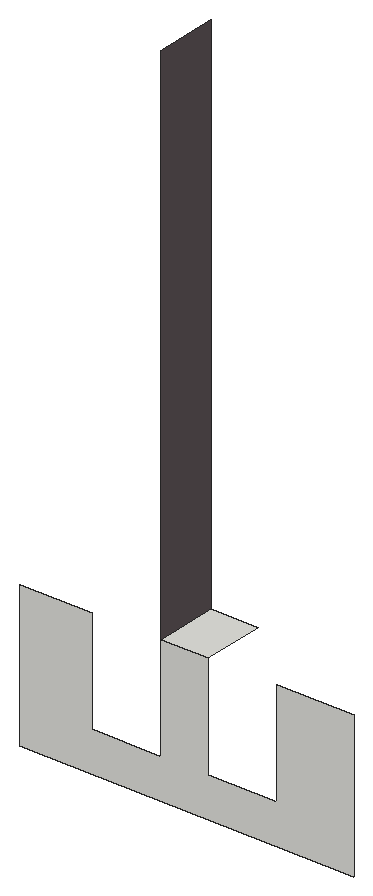
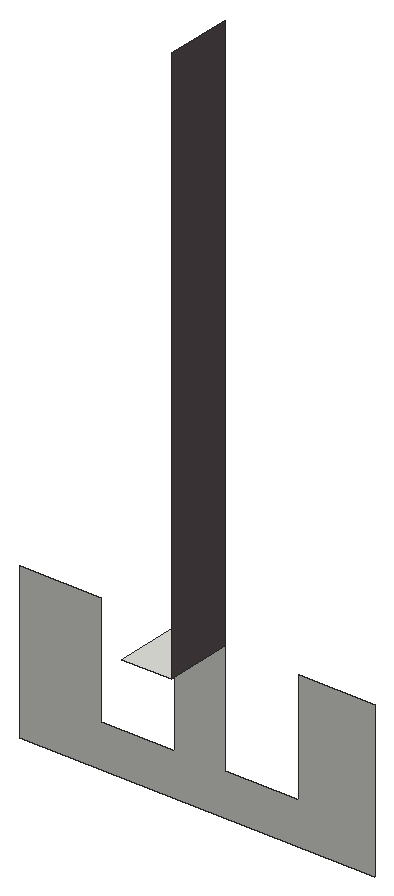
# SketchUp Ruby script. Lengths in inches.
U = 1.inch
M = Sketchup.active_model
def pt(a) = Geom::Point3d.new(a.map { |v| v * U })
def face(e, loops, mat)
  f = e.add_face(loops[0].map { |a| pt(a) })
  loops[1..].each { |l| e.add_face(l.map { |a| pt(a) }).erase! }
  f.material = f.back_material = mat if mat
  f
end
# faces: each face lists its corners as indices into pts; further lists are holes
def faces(e, pts, list, mat = nil) = list.each { |f| face(e, (f[0].is_a?(Array) ? f : [f]).map { |l| l.map { |i| pts[i] } }, mat) }
# xy, xz, yz: faces in a plane at the given z, y or x. An outline is a flat list of corners, or four numbers for a rectangle; further outlines are holes
def ring(l) = l.size == 4 ? [[l[0], l[1]], [l[2], l[1]], [l[2], l[3]], [l[0], l[3]]] : l.each_slice(2).to_a
def flat(e, list, mat, &to3) = list.each { |f| face(e, (f[0].is_a?(Array) ? f : [f]).map { |l| ring(l).map { |u, v| to3.(u, v) } }, mat) }
def xy(e, z, list, mat = nil) = flat(e, list, mat) { |x, y| [x, y, z] }
def xz(e, y, list, mat = nil) = flat(e, list, mat) { |x, z| [x, y, z] }
def yz(e, x, list, mat = nil) = flat(e, list, mat) { |y, z| [x, y, z] }
def lines(e, pts, list) = list.each { |a, b| e.add_line(pt(pts[a]), pt(pts[b])) }
# prism: a flat outline (further loops are holes) pulled along v
def prism(e, loops, v, mat = nil)
  f = face(e, loops, mat); d = Geom::Vector3d.new(v.map { |x| x * U })
  f.pushpull(f.normal.samedirection?(d) ? d.length : -d.length)
end
def box(e, o, s, mat = nil) = prism(e, [[o, [o[0] + s[0], o[1], o[2]], [o[0] + s[0], o[1] + s[1], o[2]], [o[0], o[1] + s[1], o[2]]]], [0, 0, s[2]], mat)
def at(x, y, z, deg = 0) = Geom::Transformation.translation(pt([x, y, z])) * Geom::Transformation.rotation(ORIGIN, Z_AXIS, deg.degrees)
def axes(o, x, y, z) = Geom::Transformation.new([*x, 0, *y, 0, *z, 0, *pt(o).to_a, 1])
def part(name) = M.definitions.add(name)
# library, detail: a bought-in or finely detailed component or shape, given as its bounding box
def library(name, o, s) = part(name).tap { |d| box(d.entities, o, s) }
def detail(e, o, s) = box(e.add_group.entities, o, s)
def put(e, d, t, mat = nil) = e.add_instance(d, t).tap { |i| i.material = mat if mat }
def group(e, t, mat = nil) = e.add_group.tap { |g| g.transformation = t; g.material = mat if mat }.entities
root = M.entities
M.materials.add("[Asphalt New]").color = [91, 82, 84]
xy(root,24.68,[[339.17,92.3,342.12,96.24]])
xz(root,92.3,[[330.33,15.61,351.27,15.61,351.27,24.68,346.48,24.68,346.48,18.11,342.12,18.11,342.12,24.68,339.17,24.68,339.17,18.11,334.81,18.11,334.81,24.68,330.33,24.68]])
yz(root,339.17,[[92.3,24.68,96.24,57.8125]],"[Asphalt New]")
